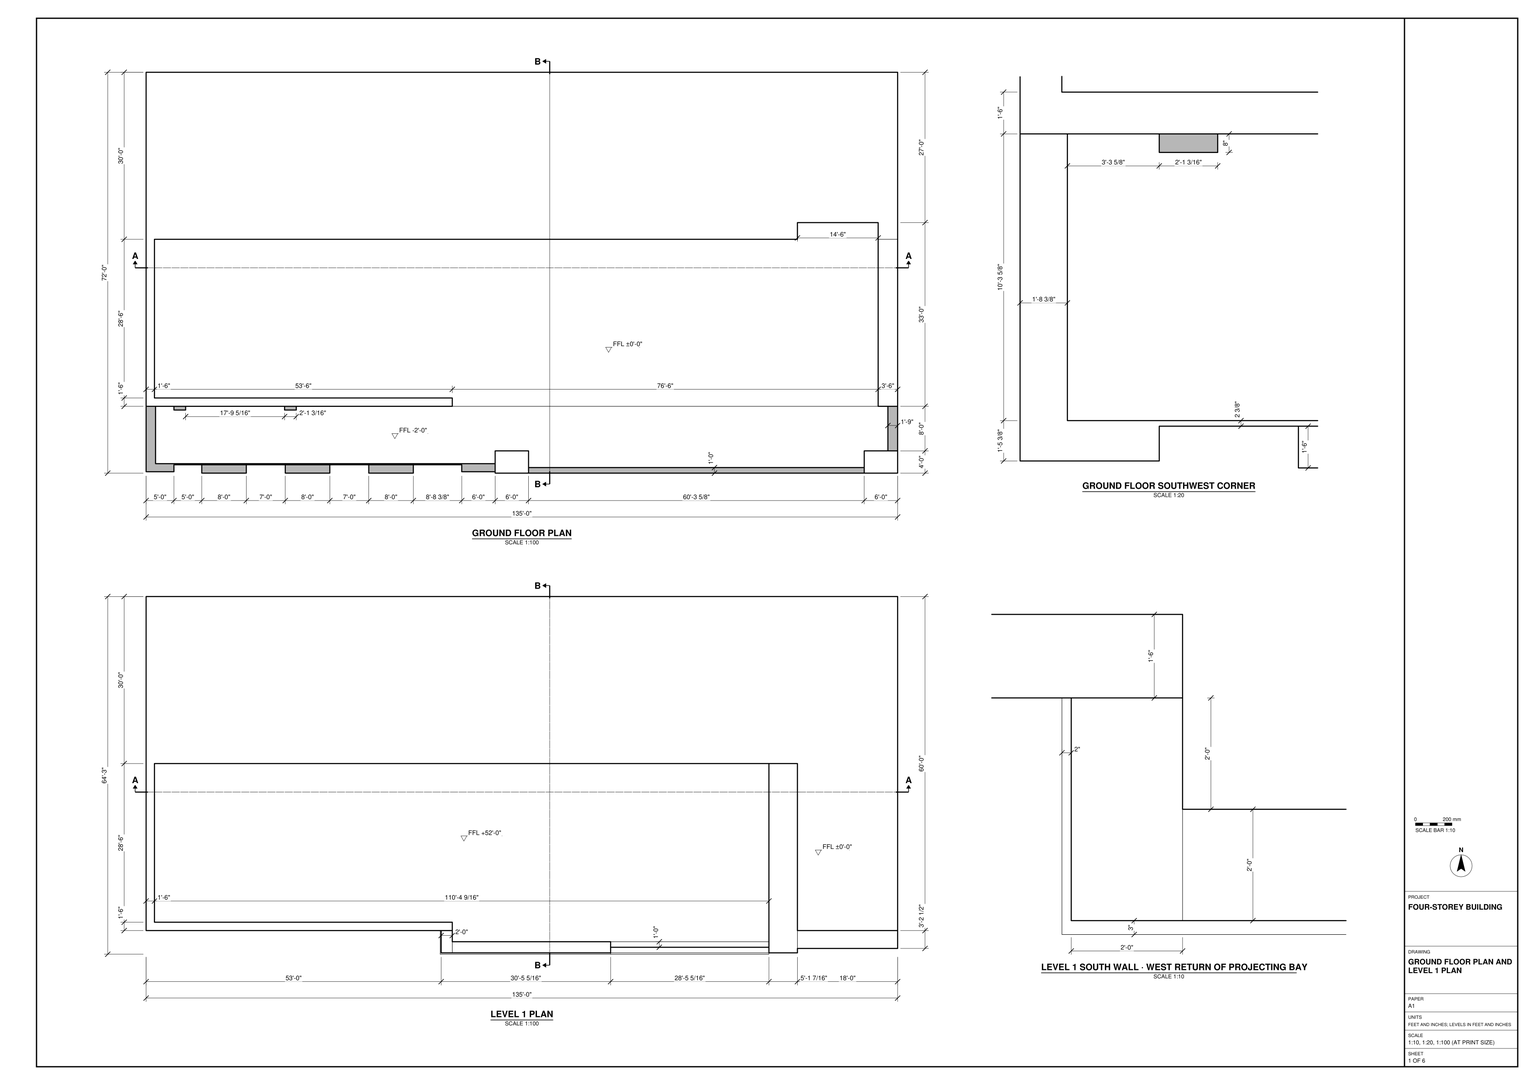
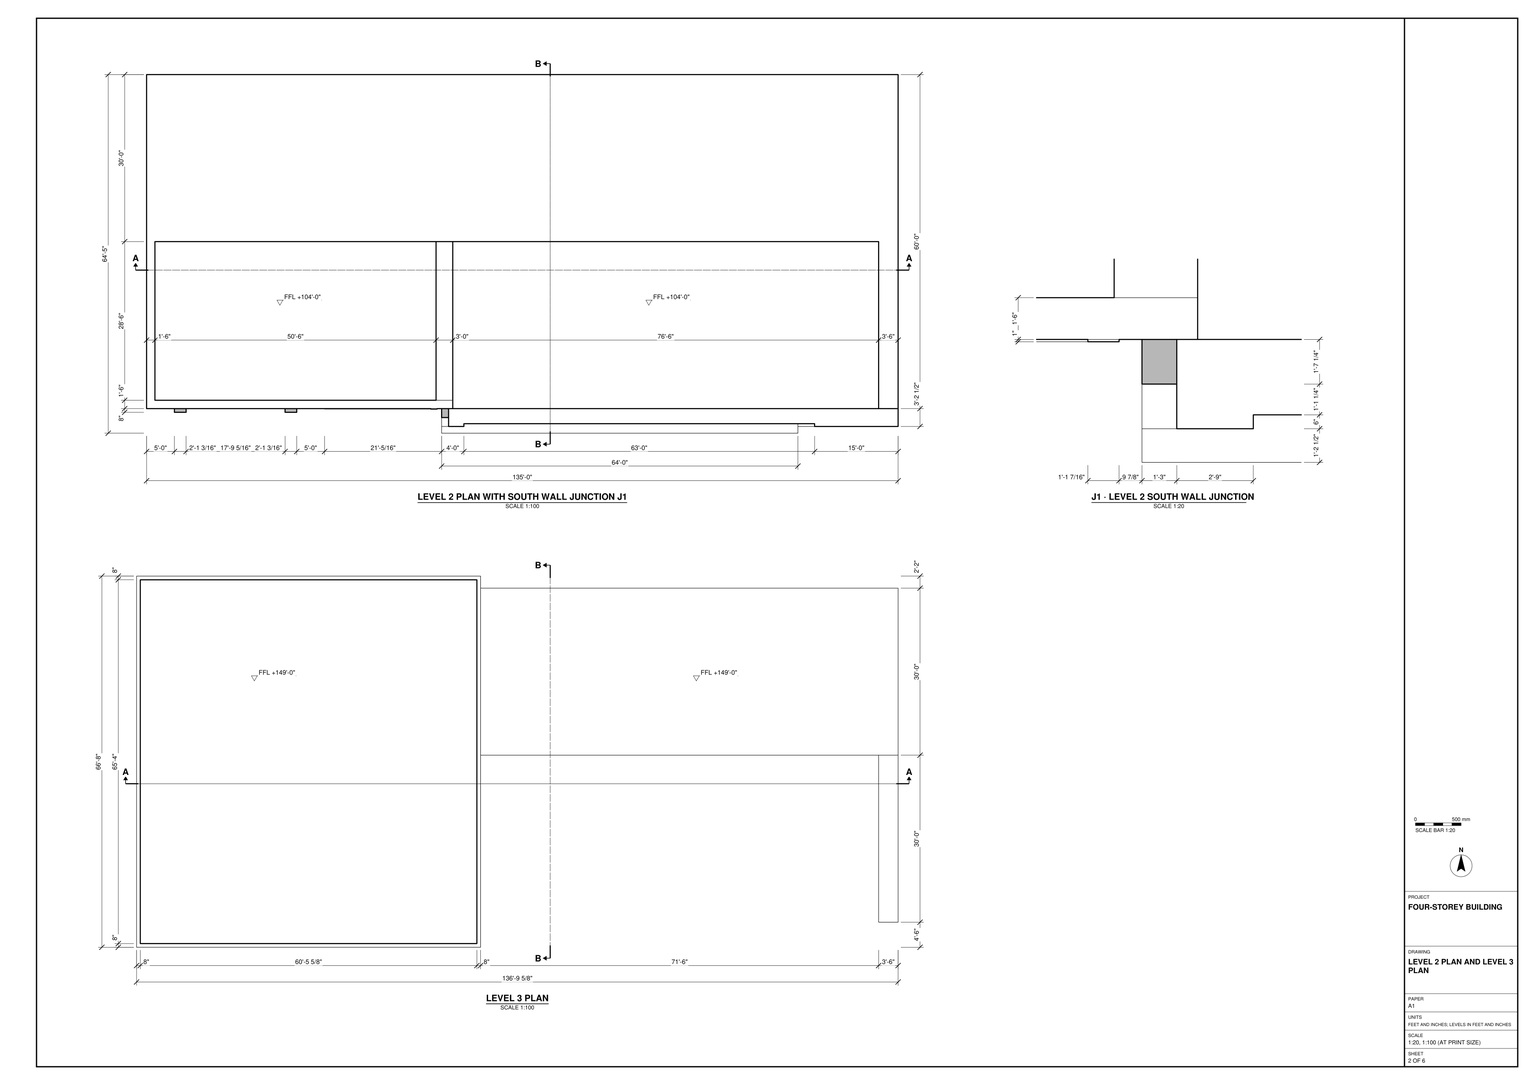
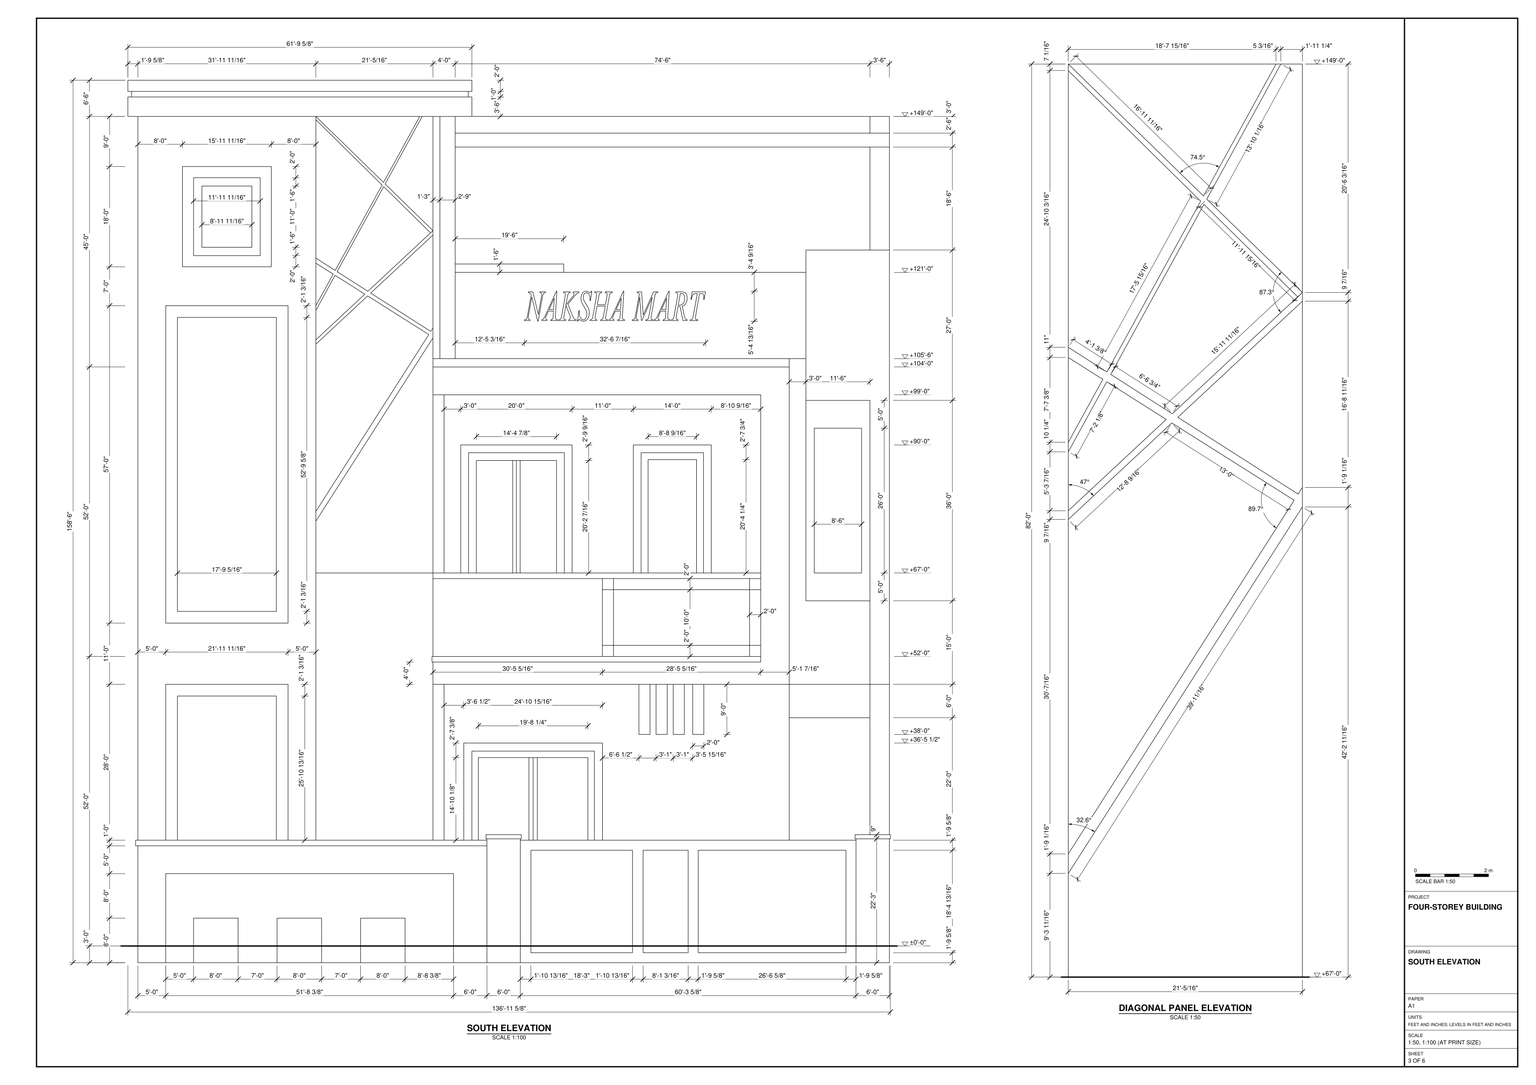
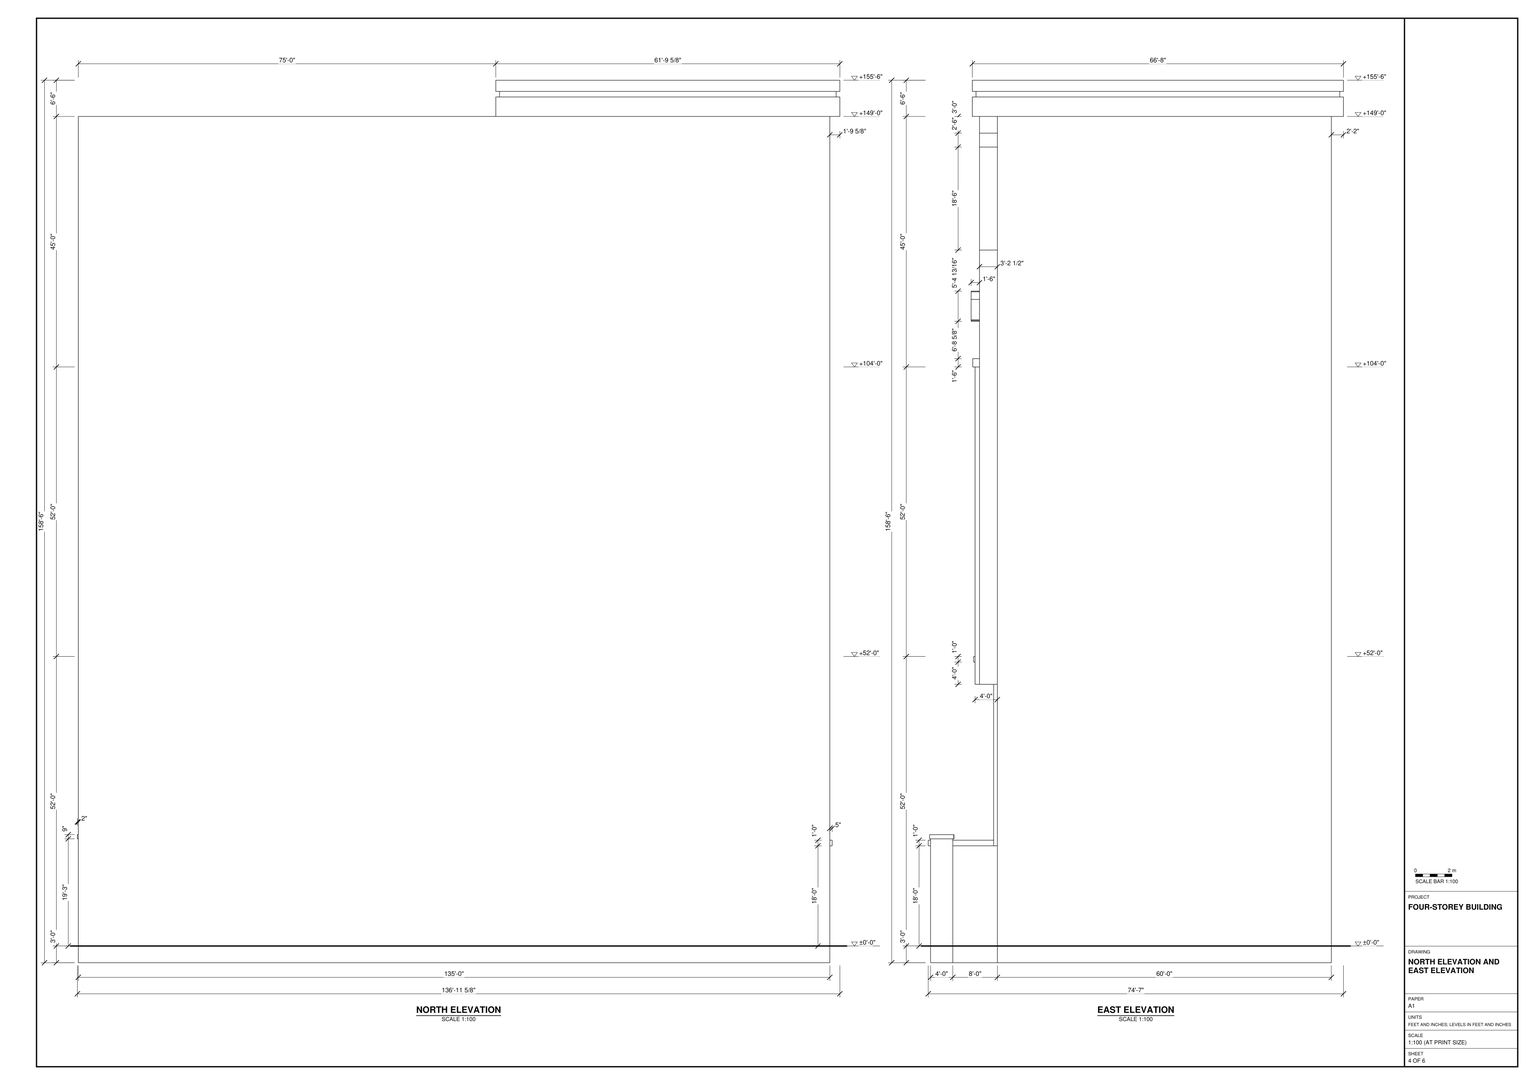
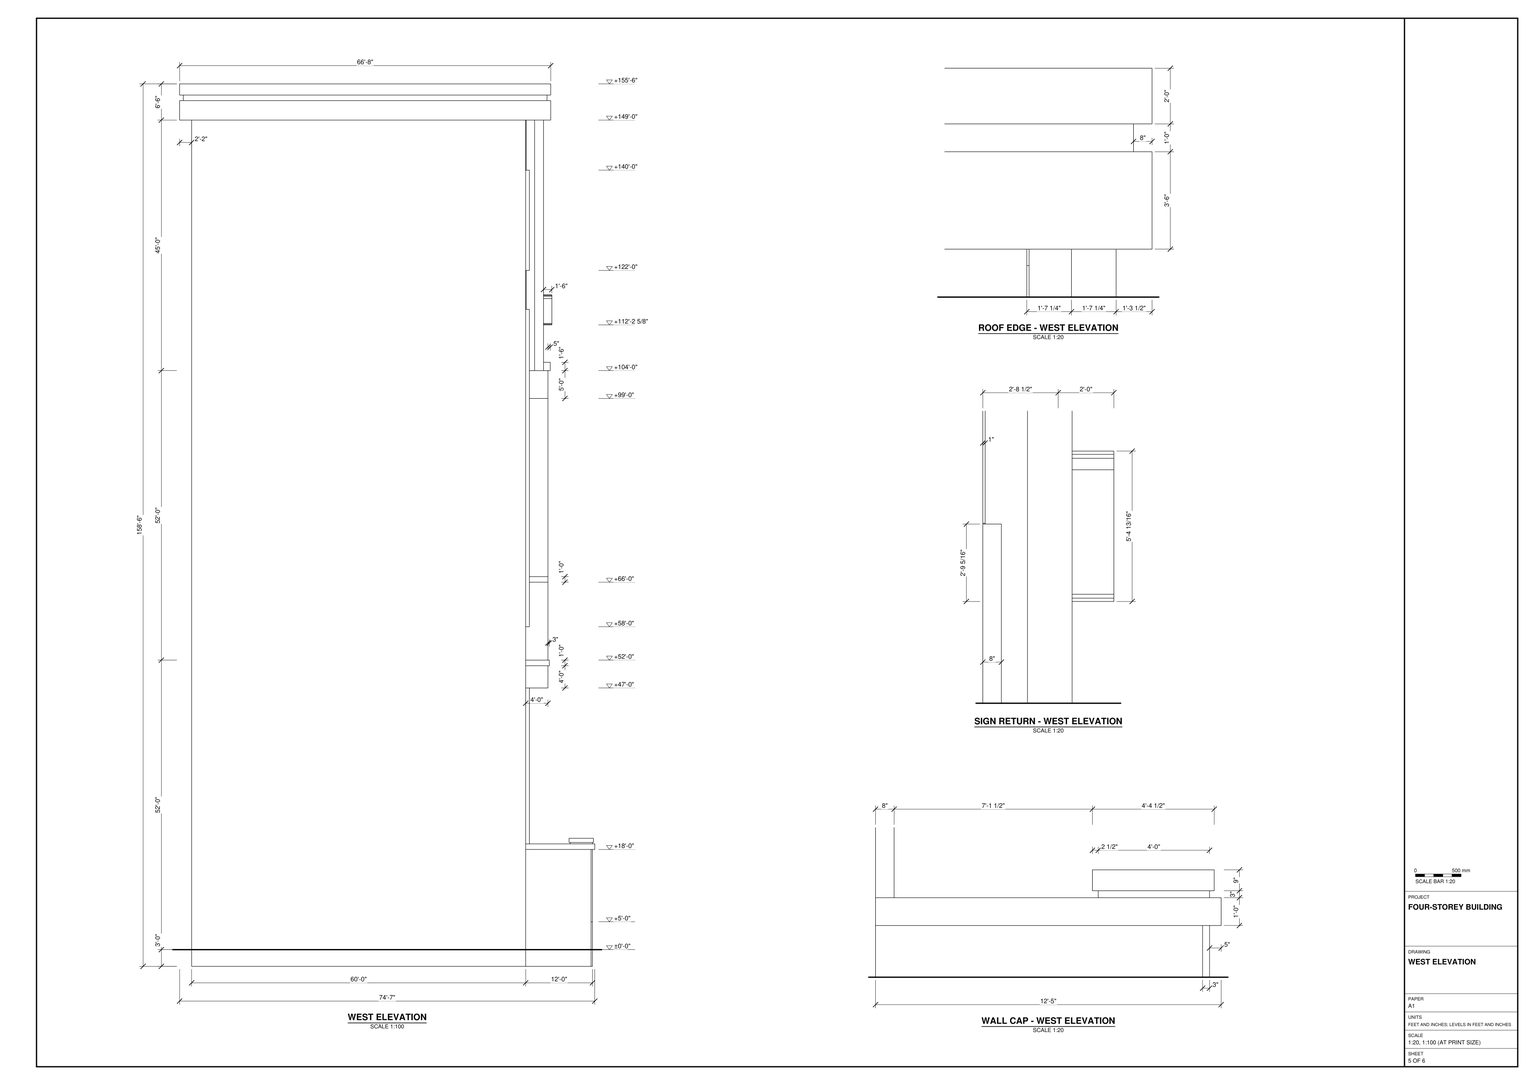
Build the four-storey building in SketchUp from task_files/diagram_01.pdf. Work in feet and inches. The overall model must measure 136'-11 5/8" east to west, 74'-7" north to south and 158'-6" high. Set the ground floor at ±0'-0" and the successive levels at +52'-0", +104'-0" and +149'-0".

Follow each floor plan separately: the slab edges and south wall change position between levels. Model the walls to their drawn thicknesses, using the enlarged details for the southwest corner, the west return of the projecting bay and the upper south wall junction. On the south elevation, form the stacked framed openings at the west, the adjacent panel with intersecting diagonal strips, and the projecting bay with its divided front and framed openings behind it. Include the entrance below the bay, the short vertical fins beside it, the sign panel above the bay and the narrow framed panel at the east. Model the low front wall with its piers and rectangular bays. Finish the roof with the raised, banded cap over the western portion and the horizontal edge extending east.

Keep walls, slabs and roof elements in separate groups or components. Group each furniture or joinery piece separately if shown, and use components for repeated parts. Any decor or loose items shown may be suitable library components. Save one SketchUp model as output_files/four_storey_building_with_its_projecting_south_bay.skp.

# SketchUp Ruby script. Lengths in inches.
U = 1.inch
M = Sketchup.active_model
def pt(a) = Geom::Point3d.new(a.map { |v| v * U })
def face(e, loops, mat)
  f = e.add_face(loops[0].map { |a| pt(a) })
  loops[1..].each { |l| e.add_face(l.map { |a| pt(a) }).erase! }
  f.material = f.back_material = mat if mat
  f
end
# faces: each face lists its corners as indices into pts; further lists are holes
def faces(e, pts, list, mat = nil) = list.each { |f| face(e, (f[0].is_a?(Array) ? f : [f]).map { |l| l.map { |i| pts[i] } }, mat) }
# xy, xz, yz: faces in a plane at the given z, y or x. An outline is a flat list of corners, or four numbers for a rectangle; further outlines are holes
def ring(l) = l.size == 4 ? [[l[0], l[1]], [l[2], l[1]], [l[2], l[3]], [l[0], l[3]]] : l.each_slice(2).to_a
def flat(e, list, mat, &to3) = list.each { |f| face(e, (f[0].is_a?(Array) ? f : [f]).map { |l| ring(l).map { |u, v| to3.(u, v) } }, mat) }
def xy(e, z, list, mat = nil) = flat(e, list, mat) { |x, y| [x, y, z] }
def xz(e, y, list, mat = nil) = flat(e, list, mat) { |x, z| [x, y, z] }
def yz(e, x, list, mat = nil) = flat(e, list, mat) { |y, z| [x, y, z] }
def lines(e, pts, list) = list.each { |a, b| e.add_line(pt(pts[a]), pt(pts[b])) }
# prism: a flat outline (further loops are holes) pulled along v
def prism(e, loops, v, mat = nil)
  f = face(e, loops, mat); d = Geom::Vector3d.new(v.map { |x| x * U })
  f.pushpull(f.normal.samedirection?(d) ? d.length : -d.length)
end
def box(e, o, s, mat = nil) = prism(e, [[o, [o[0] + s[0], o[1], o[2]], [o[0] + s[0], o[1] + s[1], o[2]], [o[0], o[1] + s[1], o[2]]]], [0, 0, s[2]], mat)
def at(x, y, z, deg = 0) = Geom::Transformation.translation(pt([x, y, z])) * Geom::Transformation.rotation(ORIGIN, Z_AXIS, deg.degrees)
def axes(o, x, y, z) = Geom::Transformation.new([*x, 0, *y, 0, *z, 0, *pt(o).to_a, 1])
def part(name) = M.definitions.add(name)
# library, detail: a bought-in or finely detailed component or shape, given as its bounding box
def library(name, o, s) = part(name).tap { |d| box(d.entities, o, s) }
def detail(e, o, s) = box(e.add_group.entities, o, s)
def put(e, d, t, mat = nil) = e.add_instance(d, t).tap { |i| i.material = mat if mat }
def group(e, t, mat = nil) = e.add_group.tap { |g| g.transformation = t; g.material = mat if mat }.entities
root = M.entities
M.materials.add("[0009_Linen]").color = [250, 240, 230]
M.materials.add("[0011_Seashell]").color = [214, 205, 199]
M.materials.add("[0011_Seashell]1").color = [221, 213, 207]
M.materials.add("[0011_Seashell]2").color = [219, 210, 204]
M.materials.add("[0013_LightCoral]").color = [255, 136, 136]
M.materials.add("[0013_LightCoral]1").color = [240, 128, 128]
M.materials.add("[0021_DarkRed]").color = [66, 0, 0]
M.materials.add("[0021_DarkRed]1").color = [43, 0, 0]
M.materials.add("[0097_DeepSkyBlue]").color = [0, 191, 255]
M.materials.add("[0133_Gray]").color = [128, 128, 128]
M.materials.add("[0136_Charcoal]").color = [35, 35, 35]
M.materials.add("[0137_Black]").color = [33, 33, 33]
M.materials.add("[0137_Black]1").color = [30, 30, 30]
M.materials.add("[Cladding Siding Tan]").color = [204, 97, 57]
M.materials.add("[Cladding Stucco White]").color = [211, 211, 211]
M.materials.add("[Granite Brown]").color = [126, 104, 91]
M.materials.add("[Granite Dark Gray]").color = [69, 68, 68]
M.materials.add("[Granite Dark Gray]1").color = [69, 68, 68]
M.materials.add("[Translucent Glass Blue]").color = [100, 149, 237]
M.materials["[Translucent Glass Blue]"].alpha = 0.5
M.materials.add("[Translucent Glass Gray]").color = [128, 128, 128]
M.materials["[Translucent Glass Gray]"].alpha = 0.5
M.materials.add("[Translucent Glass Tinted]").color = [8, 201, 241]
M.materials["[Translucent Glass Tinted]"].alpha = 0.48
M.materials.add("[White Tile Black Accent]").color = [110, 110, 110]
M.materials.add("[Wood Cherry Original]").color = [127, 72, 35]
M.materials.add("[Wood Cherry Original]1").color = [130, 73, 35]
M.materials.add("[Wood Veneer 01]").color = [120, 70, 37]
c1 = part("NAKSHA MART")
prism(c1.entities,[[[14.86,35.11,0],[25.47,8.2,0],[31.22,28.3,0],[31.92,32.15,0],[31.76,32.99,0],[31.27,33.62,0],[30.32,34.02,0],[28.81,34.15,0],[28.18,34.18,0],[28.46,35.11,0],[39.49,35.11,0],[39.19,34.18,0],[36.63,33.82,0],[35.59,33.22,0],[34.86,32.46,0],[34.04,30.82,0],[33.22,28.3,0],[25.14,0,0],[24.23,0,0],[12.81,28.96,0],[6.71,7.57,0],[6.03,3.85,0],[6.18,3,0],[6.65,2.39,0],[7.69,1.98,0],[9.59,1.72,0],[9.34,0.78,0],[-1.44,0.78,0],[-1.09,1.72,0],[1.62,2.08,0],[2.53,2.6,0],[3.16,3.27,0],[3.94,4.9,0],[4.81,7.57,0],[11.62,31.44,0],[10.6,32.72,0],[9.51,33.53,0],[8.07,33.98,0],[6,34.18,0],[6.28,35.11,0]]],[0,0,24])
prism(c1.entities,[[[61.29,35.9,0],[58.68,7.34,0],[58.48,4.71,0],[58.86,3.16,0],[60.16,2.08,0],[62.9375,1.72,0],[62.66,0.78,0],[49.14,0.78,0],[49.42,1.72,0],[50,1.72,0],[51.49,1.9,0],[52.68,2.43,0],[53.34,3.07,0],[53.82,4.03,0],[54.35,7.72,0],[54.76,12.08,0],[44.9375,12.08,0],[41.44,7.34,0],[39.95,5.05,0],[39.65,3.75,0],[39.81,2.99,0],[40.3,2.35,0],[41.18,1.91,0],[42.48,1.72,0],[42.2,0.78,0],[32.05,0.78,0],[32.33,1.72,0],[34.09,2.07,0],[35.63,2.97,0],[37.41,4.82,0],[39.9,8,0],[60.41,35.9,0]],[[56.28,27.47,0],[46.33,13.92,0],[54.96,13.92,0]]],[0,0,24])
prism(c1.entities,[[[82.81,20.3,0],[91.32,7.16,0],[93.4,4.3,0],[95.09,2.7,0],[96.82,1.97,0],[99.01,1.72,0],[98.73,0.78,0],[84.1,0.78,0],[84.33,1.72,0],[85.82,2.02,0],[86.8,2.56,0],[87.34,3.26,0],[87.52,4.05,0],[87.27,5.52,0],[85.8,8,0],[78.84,18.91,0],[75.47,7.54,0],[74.63,3.875,0],[74.81,3.03,0],[75.34,2.41,0],[76.57,1.98,0],[78.84,1.72,0],[78.43,0.78,0],[64.86,0.78,0],[65.19,1.72,0],[67.85,2.08,0],[69.34,3.24,0],[70.96,7.54,0],[77.01,28.28,0],[77.7,32.1,0],[77.53,32.99,0],[77.05,33.65,0],[76.1,34.04,0],[74.53,34.18,0],[74.03,34.18,0],[74.33,35.11,0],[87.22,35.11,0],[86.96,34.18,0],[84.58,33.82,0],[83.64,33.22,0],[82.99,32.46,0],[81.49,28.28,0],[78.84,19.47,0],[91.04,28.66,0],[93.05,30.29,0],[94.23,31.54,0],[94.68,32.73,0],[94.22,33.62,0],[92.78,34.18,0],[93.04,35.11,0],[104.03,35.11,0],[103.8,34.18,0],[100.77,33.38,0],[98.25,32.03,0],[93.32,28.28,0]]],[0,0,24])
prism(c1.entities,[[[101.19,0,0],[104.03,12.73,0],[104.89,12.73,0],[104.71,9.67,0],[104.85,8.02,0],[105.26,6.53,0],[105.95,5.19,0],[106.92,4.03,0],[108.12,3.07,0],[109.48,2.39,0],[111.01,1.98,0],[112.71,1.85,0],[114.27,1.98,0],[115.625,2.36,0],[116.79,2.99,0],[117.75,3.89,0],[119.04,6.08,0],[119.47,8.58,0],[119.27,10.23,0],[118.68,11.72,0],[116.5,14.62,0],[112.33,19.11,0],[109.11,22.89,0],[108.24,24.99,0],[107.95,27.19,0],[108.12,28.92,0],[108.62,30.53,0],[109.46,32,0],[110.63,33.34,0],[112.07,34.46,0],[113.7,35.26,0],[115.51,35.74,0],[117.52,35.9,0],[120.2,35.62,0],[123.0625,34.61,0],[124.68,33.97,0],[125.47,33.9,0],[126.73,34.28,0],[127.97,35.9,0],[128.9375,35.9,0],[126.3,24.51,0],[125.44,24.51,0],[125.54,26.96,0],[125.42,28.42,0],[125.04,29.75,0],[124.41,30.93,0],[123.52,31.97,0],[122.43,32.83,0],[121.17,33.4375,0],[118.18,33.92,0],[115.79,33.54,0],[113.9,32.38,0],[112.66,30.72,0],[112.25,28.81,0],[112.52,27.08,0],[113.3,25.43,0],[115.04,23.32,0],[118.14,20.19,0],[121.26,16.96,0],[123.04,14.52,0],[123.875,12.41,0],[124.15,10.18,0],[123.81,7.61,0],[122.77,5.125,0],[121.09,2.96,0],[118.81,1.34,0],[116.11,0.34,0],[113.16,0,0],[110.33,0.28,0],[106.125,1.65,0],[104.48,2.03,0],[103.15,1.52,0],[102.15,0,0]]],[0,0,24])
prism(c1.entities,[[[139.54,19.8,0],[155.39,19.8,0],[157.9,28.28,0],[158.61,32.125,0],[158.29,33.25,0],[157.32,33.95,0],[154.73,34.18,0],[154.99,35.11,0],[168.81,35.11,0],[168.51,34.18,0],[165.9,33.82,0],[164.84,33.22,0],[164.1,32.46,0],[163.26,30.82,0],[162.41,28.28,0],[156.35,7.54,0],[155.59,3.85,0],[155.76,3,0],[156.27,2.39,0],[157.4,1.98,0],[159.47,1.72,0],[159.19,0.78,0],[145.82,0.78,0],[146.18,1.72,0],[148.81,2.08,0],[149.68,2.59,0],[150.28,3.24,0],[151.9,7.54,0],[154.99,18.05,0],[139.0625,18.05,0],[135.95,7.54,0],[135.22,3.85,0],[135.38,3,0],[135.875,2.39,0],[137,1.98,0],[139.0625,1.72,0],[138.86,0.78,0],[125.39,0.78,0],[125.72,1.72,0],[128.38,2.08,0],[129.875,3.24,0],[131.49,7.54,0],[137.57,28.28,0],[138.3,32.125,0],[137.99,33.25,0],[137,33.95,0],[134.38,34.18,0],[134.68,35.11,0],[148.23,35.11,0],[147.95,34.18,0],[145.44,33.82,0],[144.41,33.23,0],[143.7,32.48,0],[142.9,30.875,0],[142.03,28.28,0]]],[0,0,24])
prism(c1.entities,[[[190.91,35.9,0],[188.3,7.34,0],[188.1,4.71,0],[188.48,3.16,0],[189.78,2.08,0],[192.56,1.72,0],[192.28,0.78,0],[178.76,0.78,0],[179.04,1.72,0],[179.62,1.72,0],[181.11,1.9,0],[182.3,2.43,0],[182.96,3.07,0],[183.44,4.03,0],[183.97,7.72,0],[184.38,12.08,0],[174.56,12.08,0],[171.0625,7.34,0],[169.57,5.05,0],[169.27,3.75,0],[169.43,2.99,0],[169.92,2.35,0],[170.8,1.91,0],[172.1,1.72,0],[171.82,0.78,0],[161.67,0.78,0],[161.95,1.72,0],[163.71,2.07,0],[165.25,2.97,0],[167.03,4.82,0],[169.52,8,0],[190.03,35.9,0]],[[185.9,27.47,0],[175.95,13.92,0],[184.58,13.92,0]]],[0,0,24])
prism(c1.entities,[[[225.27,35.11,0],[228.43,7.47,0],[248.35,35.11,0],[256.73,35.11,0],[256.73,34.18,0],[253.52,33.82,0],[252.72,33.33,0],[251.99,32.51,0],[251.26,31.0625,0],[250.48,28.71,0],[244.125,6.9375,0],[243.57,3.95,0],[243.74,3.08,0],[244.25,2.46,0],[245.49,1.91,0],[247.29,1.72,0],[247.9,1.72,0],[247.67,0.78,0],[233.22,0.78,0],[233.47,1.72,0],[234.15,1.72,0],[235.85,1.86,0],[237.09,2.28,0],[237.83,2.86,0],[238.49,3.81,0],[240.23,8.81,0],[245.9,28.71,0],[225.875,0.78,0],[224.86,0.78,0],[221.65,28.71,0],[215.52,7.47,0],[214.73,3.82,0],[214.91,3,0],[215.42,2.39,0],[216.59,1.98,0],[218.73,1.72,0],[218.46,0.78,0],[207.14,0.78,0],[207.42,1.72,0],[208.1,1.72,0],[210.26,2.04,0],[211.72,2.99,0],[212.55,4.43,0],[213.42,6.9375,0],[220.89,32.53,0],[219.29,33.7,0],[216.48,34.18,0],[216.73,35.11,0]]],[0,0,24])
prism(c1.entities,[[[278.73,35.9,0],[276.125,7.34,0],[275.92,4.71,0],[276.3,3.16,0],[277.61,2.08,0],[280.38,1.72,0],[280.1,0.78,0],[266.58,0.78,0],[266.86,1.72,0],[267.44,1.72,0],[268.9375,1.9,0],[270.125,2.43,0],[270.78,3.07,0],[271.27,4.03,0],[271.8,7.72,0],[272.2,12.08,0],[262.38,12.08,0],[258.89,7.34,0],[257.39,5.05,0],[257.09,3.75,0],[257.25,2.99,0],[257.75,2.35,0],[258.62,1.91,0],[259.92,1.72,0],[259.65,0.78,0],[249.49,0.78,0],[249.77,1.72,0],[251.53,2.07,0],[253.08,2.97,0],[254.86,4.82,0],[257.34,8,0],[277.85,35.9,0]],[[273.72,27.47,0],[263.77,13.92,0],[272.41,13.92,0]]],[0,0,24])
prism(c1.entities,[[[305.24,0.78,0],[299.75,17.47,0],[295.8,17.85,0],[292.84,7.47,0],[292.25,4.05,0],[292.4375,3.1,0],[292.99,2.38,0],[294.03,1.99,0],[296.03,1.72,0],[295.8,0.78,0],[282.51,0.78,0],[282.78,1.72,0],[285.32,2.1,0],[286.22,2.61,0],[286.84,3.27,0],[287.66,4.91,0],[288.53,7.47,0],[294.53,28.2,0],[295.14,31.42,0],[294.9,32.49,0],[294.19,33.39,0],[293.03,33.99,0],[291.47,34.18,0],[291.77,35.11,0],[302.96,35.11,0],[305.58,34.98,0],[307.8,34.58,0],[309.625,33.92,0],[311.0625,32.99,0],[312.15,31.84,0],[312.92,30.53,0],[313.39,29.04,0],[313.54,27.39,0],[313.39,25.77,0],[312.91,24.22,0],[312.11,22.74,0],[311,21.33,0],[309.61,20.08,0],[307.98,19.09,0],[306.12,18.34,0],[304.03,17.85,0],[307.37,7.8,0],[308.58,4.75,0],[309.8,2.99,0],[311.39,2.11,0],[313.72,1.72,0],[313.44,0.78,0]],[[296.23,19.29,0],[299.11,19.0625,0],[301.18,19.21,0],[303.01,19.67,0],[304.62,20.42,0],[306,21.48,0],[307.11,22.76,0],[307.9,24.19,0],[308.375,25.77,0],[308.53,27.49,0],[308.14,29.97,0],[306.95,31.8,0],[304.97,32.92,0],[302.2,33.29,0],[300.28,33.09,0]]],[0,0,24])
prism(c1.entities,[[[322.96,35.11,0],[349.04,35.11,0],[346.23,26,0],[345.27,26,0],[345.75,29.57,0],[345.46,31.19,0],[344.61,32.35,0],[343.07,32.89,0],[340.18,33.0625,0],[337.47,33.0625,0],[330.68,9.42,0],[329.39,3.92,0],[329.59,3.05,0],[330.2,2.34,0],[331.32,1.875,0],[333.0625,1.72,0],[334.23,1.72,0],[333.92,0.78,0],[318.99,0.78,0],[319.27,1.72,0],[319.92,1.72,0],[321.67,1.88,0],[322.96,2.35,0],[323.66,2.96,0],[324.29,3.91,0],[325.95,8.68,0],[333.0625,33.0625,0],[331.01,33.0625,0],[328.34,32.875,0],[326.24,32.3,0],[324.6,31.375,0],[323.32,30.1,0],[322.3,28.35,0],[321.49,26,0],[320.56,26,0]]],[0,0,24])
xy(root,-12,[[774,5,774,8,702,8,702,23,81.6,23,81.6,8,21.6,8,21.6,149,1641.6,149,1641.6,5],[21.6,149,1641.6,869]])
xy(root,-12,[[141.6,5,237.6,23],[321.6,5,417.6,23],[501.6,5,597.6,23]],"[0097_DeepSkyBlue]")
xy(root,0,[[81.6,141,106.8,149],[320.09,141,345.29,149]])
xy(root,0,[[846,17,1569.6,17,1569.6,53,1620.6,53,1620.6,149,345.29,149,345.29,141,320.09,141,320.09,149,106.8,149,106.8,141,81.6,141,81.6,149,42,149,42,25.4,774,25.4,774,53,846,53]],"[Granite Dark Gray]1")
xy(root,24,[[681.6,149,1599.6,149,1599.6,545,1425.6,545,1425.6,509,39.6,509,39.6,167,681.6,167]],"[Granite Dark Gray]")
xy(root,84,[[141.6,5,237.6,23],[321.6,5,417.6,23],[501.6,5,597.6,23]],"[0097_DeepSkyBlue]")
xy(root,144,[[741.6,509,1005.6,514]])
xy(root,157.875,[[755.47,509,864.6,514],[882.6,509,991.73,514]])
xy(root,180,[[81.6,8,702,23]],"[0011_Seashell]1")
xy(root,240,[[1620.6,53,1641.6,149]],"[0011_Seashell]")
xy(root,240,[[16.6,0,16.6,149,21.6,149,21.6,8,774,8,774,0]],"[0011_Seashell]1")
xy(root,252,[[846,5,1569.6,17]],"[0009_Linen]")
xy(root,252,[[16.6,0,774,0,774,25.4,42,25.4,42,149,16.6,149]],"[0011_Seashell]1")
xy(root,255,[[[772,3,848,55.5],[774,5,846,53]],[1567.6,3,1567.6,53,1569.6,53,1569.6,5,1641.6,5,1641.6,53,1567.6,53,1567.6,55,1643.6,55,1643.6,3],[774,5,846,53],[1569.6,5,1641.6,53]])
xy(root,264,[[772,3,848,55.5],[1567.6,3,1643.6,55]])
xy(root,430.125,[[755.47,509,864.6,514],[882.6,509,991.73,514]])
xy(root,444,[[741.6,509,1005.6,514]])
xy(root,516,[[1425.6,149,1599.6,545]],"[0137_Black]")
xy(root,562.8,[[106.8,141,320.09,149]])
xy(root,588,[[81.6,141,345.29,149]])
xy(root,588,[[657.6,101,657.6,149,681.6,149,681.6,167,39.6,167,39.6,509,1425.6,509,1425.6,101]],"[0011_Seashell]")
xy(root,588,[[1425.6,110.5,1641.6,149]],"[0137_Black]")
xy(root,636,[[655.6,98,655.6,149,657.6,149,657.6,101,1364.16,101,1364.16,98]],"[Wood Cherry Original]")
xy(root,648,[[657.6,101,681.6,149],[681.6,101,1022.88,125]])
xy(root,648,[[1022.88,101,1364.16,113],[1022.88,113,1364.16,125]],"[0011_Seashell]")
xy(root,648,[[681.6,125,1364.16,125,1364.16,509,39.6,509,39.6,167,681.6,167]],"[Granite Brown]")
xy(root,648,[[655.6,98,1022.88,98,1022.88,101,657.6,101,657.6,149,655.6,149],[1022.88,98,1364.16,101]],"[Wood Cherry Original]")
xy(root,712.75,[[1106.35,509,1240.85,515]])
xy(root,720,[[81.6,141,345.29,149]])
xy(root,745.2,[[106.8,141,320.09,149]])
xy(root,768,[[1461.6,110.5,1599.6,116.5]])
xy(root,816,[[1022.88,101,1364.16,113],[1022.88,113,1364.16,125]])
xy(root,828,[[657.6,101,1364.16,101,1364.16,125,681.6,125,681.6,149,657.6,149]],"[Wood Cherry Original]")
xy(root,828,[[1479.6,110.5,1581.6,121]],"[Wood Veneer 01]")
xy(root,1087.25,[[1106.35,509,1240.85,515]])
xy(root,1140,[[1479.6,110.5,1581.6,121]],"[Wood Veneer 01]")
xy(root,1200,[[1461.6,110.5,1599.6,116.5]])
xy(root,1212,[[657.6,101,657.6,149,681.6,149,681.6,167,39.6,167,39.6,509,1364.16,509,1364.16,101]],"[0011_Seashell]")
xy(root,1272,[[657.6,101,1425.6,110.5],[657.6,110.5,672.6,129.75],[657.6,129.75,672.6,149],[39.6,167,645.6,509],[645.6,167,681.6,509]])
xy(root,1272,[[681.6,149,1599.6,509]],"[Granite Brown]")
xy(root,1272,[[657.6,96,1425.6,101]],"[Wood Veneer 01]")
xy(root,1290,[[1425.6,110.5,1461.6,116.5]],"[0136_Charcoal]")
xy(root,1290,[[657.6,96,1425.6,96,1425.6,116.5,705.6,116.5,705.6,110.5,657.6,110.5]],"[Wood Veneer 01]")
xy(root,1378.8,[[106.8,141,320.09,149]])
xy(root,1404,[[81.6,141,345.29,149]])
xy(root,1476,[[705.6,116.5,939.6,149]])
xy(root,1476,[[939.6,116.5,1461.6,149]],"[0137_Black]")
xy(root,1476,[[705.6,110.5,939.6,116.5]],"[Wood Veneer 01]")
xy(root,1488,[[117.6,141,309.29,149]],"[Wood Veneer 01]")
xy(root,1494,[[705.6,110.5,939.6,149]],"[Wood Veneer 01]")
xy(root,1512,[[141.6,141,285.29,149]],"[Wood Veneer 01]")
xy(root,1524,[[1461.6,110.5,1641.6,149]],"[0013_LightCoral]")
xy(root,1680,[[141.6,141,285.29,149]],"[Wood Veneer 01]")
xy(root,1704,[[117.6,141,309.29,149]],"[Wood Veneer 01]")
xy(root,1746,[[705.6,110.5,1641.6,149],[747.6,149,778.8,509],[838.8,149,870,509],[930,149,961.2,509],[1021.2,149,1052.4,509],
  [1112.4,149,1143.6,509],[1203.6,149,1234.8,509],[1294.8,149,1326,509],[1386,149,1417.2,509],[1477.2,149,1508.4,509],
  [1568.4,149,1599.6,509]],"[Wood Veneer 01]")
xy(root,1776,[[705.6,110.5,1641.6,149],[747.6,149,778.8,509],[838.8,149,870,509],[930,149,961.2,509],[1021.2,149,1052.4,509],
  [1112.4,149,1143.6,509],[1203.6,149,1234.8,509],[1294.8,149,1326,509],[1386,149,1417.2,509],[1477.2,149,1508.4,509],
  [1568.4,149,1599.6,509]],"[Wood Veneer 01]")
xy(root,1794,[[681.6,149,705.6,509]],"[Wood Veneer 01]")
xy(root,1812,[[672.6,110.5,705.6,149],[657.6,129.75,672.6,149],[629.2,148,629.2,149,21.6,149,21.6,509,39.6,509,39.6,167,681.6,167,681.6,149,634.37,149,634.37,148],[681.6,149,705.6,167],[39.6,167,645.6,509],
  [645.6,167,681.6,509],[681.6,167,705.6,509],[21.6,509,741.6,869]])
xy(root,1812,[[1599.6,149,1641.6,509],[741.6,509,1641.6,869]],"[0011_Seashell]")
xy(root,1812,[[0,95,0,895,741.6,895,741.6,869,21.6,869,21.6,149,629.2,149,629.2,148,634.37,148,634.37,149,657.6,149,657.6,129.75,672.6,129.75,672.6,110.5,705.6,110.5,705.6,509,741.6,509,741.6,95]],"[0011_Seashell]2")
xy(root,1854,[[8,103,733.6,887]])
xy(root,1854,[[[0,95,741.6,895],[8,103,733.6,887]]],"[0011_Seashell]2")
xy(root,1866,[[8,103,733.6,887]])
xy(root,1866,[[[0,95,741.6,895],[8,103,733.6,887]]],"[0011_Seashell]2")
xy(root,1890,[[0,95,741.6,895]],"[0011_Seashell]2")
xz(root,0,[[16.6,240,774,252]],"[0011_Seashell]1")
xz(root,3,[[772,255,848,264],[1567.6,255,1643.6,264]])
xz(root,5,[[774,-12,846,255],[1569.6,-12,1641.6,255]])
xz(root,5,[[141.6,-12,237.6,84],[321.6,-12,417.6,84],[501.6,-12,597.6,84],[868.8,9.6,1087.8,230.4],[1110.6,9.6,1207.8,230.4]],"[0097_DeepSkyBlue]")
xz(root,5,[[[846,-12,1569.6,252],[1229.4,9.6,1548,230.4],[868.8,9.6,1087.8,230.4],[1110.6,9.6,1207.8,230.4]]],"[0137_Black]1")
xz(root,5,[[1229.4,9.6,1548,230.4]],"[Cladding Siding Tan]")
xz(root,8,[[21.6,-12,81.6,-12,81.6,180,702,180,702,-12,774,-12,774,240,21.6,240]],"[0011_Seashell]1")
xz(root,17,[[846,0,1569.6,252]],"[0009_Linen]")
xz(root,23,[[81.6,-12,141.6,-12,141.6,84,237.6,84,237.6,-12,321.6,-12,321.6,84,417.6,84,417.6,-12,501.6,-12,501.6,84,597.6,84,597.6,-12,702,-12,702,180,81.6,180],[141.6,-12,237.6,84],[321.6,-12,417.6,84],[501.6,-12,597.6,84]])
xz(root,25.4,[[42,0,774,252]],"[0011_Seashell]1")
xz(root,53,[[774,0,846,255],[1569.6,0,1569.6,255,1641.6,255,1641.6,240,1620.6,240,1620.6,0],[1620.6,0,1641.6,240]])
xz(root,55,[[1567.6,255,1643.6,264]])
xz(root,55.5,[[772,255,848,264]])
xz(root,95,[[0,1812,741.6,1854],[0,1866,741.6,1890]],"[0011_Seashell]2")
xz(root,96,[[657.6,1272,1425.6,1290]],"[Wood Veneer 01]")
xz(root,98,[[655.6,636,1364.16,648]],"[Wood Cherry Original]")
xz(root,101,[[657.6,636,1364.16,648]])
xz(root,101,[[657.6,588,1425.6,588,1425.6,1272,657.6,1272,657.6,1212,1364.16,1212,1364.16,636,657.6,636],[657.6,648,1022.88,816]],"[0011_Seashell]")
xz(root,101,[[657.6,816,1364.16,828]],"[Wood Cherry Original]")
xz(root,103,[[8,1854,733.6,1866]],"[0133_Gray]")
xz(root,110.5,[[1599.6,588,1641.6,588,1641.6,1524,1461.6,1524,1461.6,1200,1599.6,1200]],"[0013_LightCoral]")
xz(root,110.5,[[1425.6,588,1599.6,588,1599.6,768,1461.6,768,1461.6,1290,1425.6,1290]],"[0137_Black]")
xz(root,110.5,[[[1461.6,768,1599.6,1200],[1479.6,828,1581.6,1140]],[657.6,1272,672.6,1290],[672.6,1290,705.6,1812],[705.6,1476,939.6,1494],[705.6,1746,1641.6,1776]],"[Wood Veneer 01]")
xz(root,113,[[1046.88,648,1340.16,672]],"[0011_Seashell]")
xz(root,113,[[1022.88,648,1046.88,672],[1340.16,648,1364.16,672],[1022.88,672,1046.88,792],[1046.88,672,1340.16,792],[1340.16,672,1364.16,792],
  [1022.88,792,1046.88,816],[1046.88,792,1340.16,816],[1340.16,792,1364.16,816]],"[Translucent Glass Gray]")
xz(root,116.5,[[1461.6,768,1461.6,1476,705.6,1476,705.6,1290,1461.6,1290,1461.6,1200,1599.6,1200,1599.6,768]],"[Cladding Stucco White]")
xz(root,121,[[1479.6,828,1581.6,1140]])
xz(root,125,[[1022.88,816,1364.16,828]])
xz(root,125,[[681.6,648,1022.88,828]],"[0011_Seashell]")
xz(root,129.75,[[657.6,1272,672.6,1812]])
xz(root,141,[[81.6,0,106.8,0,106.8,562.8,320.09,562.8,320.09,0,345.29,0,345.29,588,81.6,588],[[81.6,720,345.29,1404],[106.8,745.2,320.09,1378.8]]])
xz(root,141,[[[117.6,1488,309.29,1704],[141.6,1512,285.29,1680]]],"[Wood Veneer 01]")
xz(root,148,[[405.29,939.7,657.6,1334.69,657.6,1355.75,652.98,1348.52,523.39,1431.3,657.6,1556.41,657.6,1565.84,652.52,1561.11,517.39,1435.13,451.03,1477.52,551.47,1660.76,652.52,1561.11,657.6,1565.84,554.55,1666.38,634.37,1812,629.2,1812,551.08,1669.77,405.29,1812,405.29,1804.92,548,1664.18,446.92,1480.15,405.29,1506.74,405.29,1495.74,442.55,1472.19,405.29,1404.36,405.29,1394.07,446.68,1469.58,510.84,1429.03,405.29,1330.63,405.29,1321.2,516.875,1425.22,648.74,1341.88,405.29,960.75]])
xz(root,149,[[21.6,-12,1641.6,0],[21.6,0,42,252],[81.6,0,81.6,588,345.29,588,345.29,0,320.09,0,320.09,562.8,106.8,562.8,106.8,0],[106.8,0,320.09,562.8],[657.6,0,681.6,588],
  [1620.6,0,1641.6,240],[16.6,240,21.6,252],[657.6,588,681.6,624],[1425.6,588,1425.6,1272,1641.6,1272,1641.6,624,1599.6,624,1599.6,588],[1599.6,588,1641.6,624],
  [657.6,624,681.6,648],[655.6,636,657.6,648],[657.6,648,681.6,828],[[81.6,720,345.29,1404],[106.8,745.2,320.09,1378.8]],[657.6,1272,672.6,1812],
  [672.6,1272,681.6,1812],[1599.6,1272,1641.6,1524],[[117.6,1488,309.29,1704],[141.6,1512,285.29,1680]],[[141.6,1512,285.29,1680],[159.6,1530,267.29,1662]],[747.6,1746,778.8,1776],
  [838.8,1746,870,1776],[930,1746,961.2,1776],[1021.2,1746,1052.4,1776],[1112.4,1746,1143.6,1776],[1203.6,1746,1234.8,1776],
  [1294.8,1746,1326,1776],[1386,1746,1417.2,1776],[1477.2,1746,1508.4,1776],[1568.4,1746,1599.6,1776],[1599.6,1746,1641.6,1776]])
xz(root,149,[[657.6,828,681.6,1212],[1599.6,1524,1641.6,1746],[1599.6,1776,1641.6,1812]],"[0011_Seashell]")
xz(root,149,[[[42,0,81.6,0,81.6,588,345.29,588,345.29,0,405.29,0,405.29,1812,21.6,1812,21.6,252,42,252],[81.6,720,345.29,1404],[117.6,1488,309.29,1704]]],"[0011_Seashell]2")
xz(root,149,[[1599.6,0,1620.6,0,1620.6,240,1641.6,240,1641.6,588,1599.6,588]],"[0013_LightCoral]")
xz(root,149,[[1425.6,516,1599.6,588],[681.6,1272,681.6,1794,705.6,1794,705.6,1476,1461.6,1476,1461.6,1524,1599.6,1524,1599.6,1272]],"[0137_Black]")
xz(root,149,[[405.29,0,657.6,0,657.6,636,655.6,636,655.6,648,657.6,648,657.6,828,405.29,828]],"[Cladding Stucco White]")
xz(root,149,[[681.6,0,1599.6,24]],"[Granite Dark Gray]1")
xz(root,149,[[159.6,1530,267.29,1662]],"[Translucent Glass Blue]")
xz(root,149,[[405.29,828,657.6,828,657.6,1334.69,405.29,939.7],[405.29,960.75,648.74,1341.88,516.875,1425.22,405.29,1321.2],[405.29,1330.63,510.84,1429.03,446.68,1469.58,405.29,1394.07],[652.98,1348.52,657.6,1355.75,657.6,1556.41,523.39,1431.3],[405.29,1404.36,442.55,1472.19,405.29,1495.74],
  [517.39,1435.13,652.52,1561.11,551.47,1660.76,451.03,1477.52],[446.92,1480.15,548,1664.18,405.29,1804.92,405.29,1506.74],[657.6,1565.84,657.6,1812,634.37,1812,554.55,1666.38],[551.08,1669.77,629.2,1812,405.29,1812]],"[Translucent Glass Tinted]")
xz(root,149,[[106.8,745.2,320.09,1378.8]],"[White Tile Black Accent]")
xz(root,149,[[870,1746,930,1776],[961.2,1746,1021.2,1776],[1052.4,1746,1112.4,1776],[1143.6,1746,1203.6,1776],[1234.8,1746,1294.8,1776],
  [1326,1746,1386,1776],[1417.2,1746,1477.2,1776],[1508.4,1746,1568.4,1776]],"[Wood Cherry Original]1")
xz(root,149,[[705.6,1476,939.6,1494],[705.6,1746,747.6,1776],[778.8,1746,838.8,1776]],"[Wood Veneer 01]")
xz(root,167,[[39.6,1272,645.6,1812]])
xz(root,167,[[39.6,24,681.6,588],[39.6,648,681.6,1212]],"[0011_Seashell]")
xz(root,509,[[[724.125,126.52,1023.08,461.48],[741.6,144,1005.6,444]],[39.6,588,681.6,624],[681.6,588,1425.6,624],[1364.16,648,1364.16,1212,1341.6,1212,1341.6,1248,1425.6,1248,1425.6,648],[[1089.6,696,1257.6,1104],[1106.35,712.75,1240.85,1087.25]],
  [[717.6,780,957.6,1104],[734.35,796.75,940.85,1087.25]],[39.6,1272,645.6,1812],[645.6,1272,681.6,1812],[1568.4,1746,1599.6,1776],[681.6,1794,705.6,1812]])
xz(root,509,[[[39.6,24,1425.6,24,1425.6,588,1241.54,588,1241.54,480,1217.54,480,1217.54,588,1199.6,588,1199.6,480,1175.6,480,1175.6,588,1162.6,588,1162.6,480,1138.6,480,1138.6,588,1125.6,588,1125.6,480,1101.6,480,1101.6,588,39.6,588],[724.125,126.52,1023.08,461.48]],[[39.6,648,1364.16,1212],[717.6,780,957.6,1104],[1089.6,696,1257.6,1104]],[[681.6,1272,1599.6,1272,1599.6,1746,1568.4,1746,1568.4,1776,1599.6,1776,1599.6,1812,705.6,1812,705.6,1794,681.6,1794],[747.6,1746,778.8,1776],[838.8,1746,870,1776],[930,1746,961.2,1776],[1021.2,1746,1052.4,1776],[1112.4,1746,1143.6,1776],[1203.6,1746,1234.8,1776],[1294.8,1746,1326,1776],[1386,1746,1417.2,1776],[1477.2,1746,1508.4,1776]]],"[0011_Seashell]")
xz(root,509,[[[734.35,796.75,940.85,1087.25],[751.15,813.55,924.05,1070.45]],[829.6,813.55,837.6,1070.45],[837.6,813.55,845.6,1070.45]],"[0021_DarkRed]")
xz(root,509,[[1101.6,480,1125.6,588],[1138.6,480,1162.6,588],[1175.6,480,1199.6,588],[1217.54,480,1241.54,588]],"[0021_DarkRed]1")
xz(root,509,[[755.47,157.875,864.6,430.125],[882.6,157.875,991.73,430.125]],"[Translucent Glass Gray]")
xz(root,509,[[751.15,813.55,829.6,1070.45],[845.6,813.55,924.05,1070.45]],"[Translucent Glass Tinted]")
xz(root,514,[[[741.6,144,1005.6,444],[755.47,157.875,991.73,430.125]],[864.6,157.875,873.6,430.125],[873.6,157.875,882.6,430.125]],"[0021_DarkRed]")
xz(root,515,[[[1106.35,712.75,1240.85,1087.25],[1121.33,727.73,1225.87,1072.27]]],"[0021_DarkRed]")
xz(root,515,[[1121.33,727.73,1225.87,1072.27]],"[Translucent Glass Tinted]")
xz(root,545,[[1425.6,24,1599.6,516]],"[0013_LightCoral]")
xz(root,869,[[21.6,-12,1641.6,1812]],"[0011_Seashell]1")
xz(root,887,[[8,1851.6875,733.6,1854]])
xz(root,887,[[8,1854,733.6,1866]],"[0133_Gray]")
xz(root,895,[[0,1812,741.6,1854],[0,1866,741.6,1890]],"[0011_Seashell]2")
yz(root,0,[[95,1812,895,1854],[95,1866,895,1890]],"[0011_Seashell]2")
yz(root,8,[[103,1851.6875,887,1854]])
yz(root,8,[[103,1854,887,1866]],"[0133_Gray]")
yz(root,16.6,[[0,240,149,252]],"[0011_Seashell]1")
yz(root,21.6,[[8,-12,149,240],[149,-12,869,1812]],"[0011_Seashell]1")
yz(root,39.6,[[167,588,509,624],[167,1272,509,1812]])
yz(root,39.6,[[167,24,509,588],[167,648,509,1212]],"[0011_Seashell]")
yz(root,42,[[25.4,0,149,252]],"[0011_Seashell]1")
yz(root,81.6,[[141,0,149,588],[141,720,149,1404]])
yz(root,81.6,[[8,-12,23,180]],"[0011_Seashell]1")
yz(root,106.8,[[141,0,149,562.8],[141,745.2,149,1378.8]])
yz(root,117.6,[[141,1488,149,1704]],"[Wood Veneer 01]")
yz(root,141.6,[[5,-12,23,84]],"[0097_DeepSkyBlue]")
yz(root,141.6,[[141,1512,149,1680]],"[Wood Veneer 01]")
yz(root,237.6,[[5,-12,23,84]],"[0097_DeepSkyBlue]")
yz(root,285.29,[[141,1512,149,1680]],"[Wood Veneer 01]")
yz(root,309.29,[[141,1488,149,1704]],"[Wood Veneer 01]")
yz(root,320.09,[[141,0,149,562.8],[141,745.2,149,1378.8]])
yz(root,321.6,[[5,-12,23,84]],"[0097_DeepSkyBlue]")
yz(root,345.29,[[141,0,149,588],[141,720,149,1404]])
yz(root,405.29,[[148,939.7,149,960.75],[148,1321.2,149,1330.63],[148,1394.07,149,1404.36],[148,1495.74,149,1506.74],[148,1804.92,149,1812]])
yz(root,417.6,[[5,-12,23,84]],"[0097_DeepSkyBlue]")
yz(root,501.6,[[5,-12,23,84]],"[0097_DeepSkyBlue]")
yz(root,597.6,[[5,-12,23,84]],"[0097_DeepSkyBlue]")
yz(root,645.6,[[167,1272,509,1812]])
yz(root,655.6,[[98,636,149,648]],"[Wood Cherry Original]")
yz(root,657.6,[[101,588,149,636],[101,636,149,648],[101,648,149,816],[101,1212,149,1272],[129.75,1272,129.75,1812,149,1812,149,1565.84,148,1565.84,148,1556.41,149,1556.41,149,1355.75,148,1355.75,148,1334.69,149,1334.69,149,1272],
  [148,1334.69,149,1355.75],[148,1556.41,149,1565.84]])
yz(root,657.6,[[101,816,149,828]],"[Wood Cherry Original]")
yz(root,657.6,[[96,1272,110.5,1290]],"[Wood Veneer 01]")
yz(root,672.6,[[129.75,1272,149,1812]])
yz(root,672.6,[[110.5,1272,129.75,1812]],"[Wood Veneer 01]")
yz(root,681.6,[[149,588,167,624],[149,1794,509,1812]])
yz(root,681.6,[[149,24,167,588],[125,648,149,828],[149,648,167,1212],[149,1272,509,1794]],"[0011_Seashell]")
yz(root,702,[[8,-12,23,180]],"[0011_Seashell]1")
yz(root,705.6,[[110.5,1476,149,1494],[110.5,1746,149,1776]])
yz(root,705.6,[[110.5,1290,116.5,1476],[110.5,1494,149,1746],[110.5,1776,149,1776,149,1794,509,1794,509,1812,110.5,1812]],"[Wood Veneer 01]")
yz(root,733.6,[[103,1854,887,1866]],"[0133_Gray]")
yz(root,741.6,[[509,144,514,444]])
yz(root,741.6,[[95,1812,895,1854],[95,1866,895,1890]],"[0011_Seashell]2")
yz(root,747.6,[[149,1746,509,1776]],"[Wood Veneer 01]")
yz(root,755.47,[[509,157.875,514,430.125]])
yz(root,772,[[3,255,55.5,264]])
yz(root,774,[[5,-12,8,240],[25.4,0,25.4,252,5,252,5,255,53,255,53,0],[8,0,8,240,5,240,5,252,25.4,252,25.4,0]])
yz(root,774,[[0,240,5,252]],"[0011_Seashell]1")
yz(root,778.8,[[149,1746,509,1776]],"[Wood Veneer 01]")
yz(root,838.8,[[149,1746,509,1776]],"[Wood Veneer 01]")
yz(root,846,[[17,0,53,0,53,255,5,255,5,252,17,252],[5,0,17,252]])
yz(root,848,[[3,255,55.5,264]])
yz(root,864.6,[[509,157.875,514,430.125]])
yz(root,870,[[149,1746,509,1776]],"[Wood Veneer 01]")
yz(root,882.6,[[509,157.875,514,430.125]])
yz(root,930,[[149,1746,509,1776]],"[Wood Veneer 01]")
yz(root,939.6,[[110.5,1476,149,1494]],"[Wood Veneer 01]")
yz(root,961.2,[[149,1746,509,1776]],"[Wood Veneer 01]")
yz(root,991.73,[[509,157.875,514,430.125]])
yz(root,1005.6,[[509,144,514,444]])
yz(root,1021.2,[[149,1746,509,1776]],"[Wood Veneer 01]")
yz(root,1022.88,[[101,648,113,816],[113,648,125,816]],"[0011_Seashell]")
yz(root,1052.4,[[149,1746,509,1776]],"[Wood Veneer 01]")
yz(root,1106.35,[[509,712.75,515,1087.25]])
yz(root,1112.4,[[149,1746,509,1776]],"[Wood Veneer 01]")
yz(root,1143.6,[[149,1746,509,1776]],"[Wood Veneer 01]")
yz(root,1203.6,[[149,1746,509,1776]],"[Wood Veneer 01]")
yz(root,1234.8,[[149,1746,509,1776]],"[Wood Veneer 01]")
yz(root,1240.85,[[509,712.75,515,1087.25]])
yz(root,1294.8,[[149,1746,509,1776]],"[Wood Veneer 01]")
yz(root,1326,[[149,1746,509,1776]],"[Wood Veneer 01]")
yz(root,1364.16,[[98,636,101,648],[101,648,113,816]])
yz(root,1364.16,[[113,648,113,816,125,816,125,828,101,828,101,1212,509,1212,509,648]],"[0011_Seashell]")
yz(root,1386,[[149,1746,509,1776]],"[Wood Veneer 01]")
yz(root,1417.2,[[149,1746,509,1776]],"[Wood Veneer 01]")
yz(root,1425.6,[[110.5,588,149,624],[149,588,509,624],[110.5,624,149,648],[149,648,509,1248]])
yz(root,1425.6,[[101,588,110.5,1272]],"[0011_Seashell]2")
yz(root,1425.6,[[509,24,545,516]],"[0013_LightCoral]")
yz(root,1425.6,[[149,516,509,588]],"[0137_Black]")
yz(root,1425.6,[[96,1272,110.5,1290]],"[Wood Veneer 01]")
yz(root,1461.6,[[110.5,768,116.5,1200],[110.5,1200,116.5,1290]])
yz(root,1461.6,[[110.5,1290,110.5,1524,149,1524,149,1476,116.5,1476,116.5,1290]],"[0013_LightCoral]1")
yz(root,1477.2,[[149,1746,509,1776]],"[Wood Veneer 01]")
yz(root,1479.6,[[110.5,828,121,1140]],"[Wood Veneer 01]")
yz(root,1508.4,[[149,1746,509,1776]],"[Wood Veneer 01]")
yz(root,1567.6,[[3,255,55,264]])
yz(root,1568.4,[[149,1746,509,1776]],"[Wood Veneer 01]")
yz(root,1569.6,[[17,0,17,252,5,252,5,255,53,255,53,0],[5,0,17,252]])
yz(root,1581.6,[[110.5,828,121,1140]],"[Wood Veneer 01]")
yz(root,1599.6,[[149,516,509,624],[110.5,768,116.5,1200],[149,1746,509,1776]])
yz(root,1599.6,[[149,1272,509,1746]],"[0011_Seashell]")
yz(root,1599.6,[[149,1776,509,1812]],"[0011_Seashell]2")
yz(root,1599.6,[[149,24,545,516]],"[0013_LightCoral]")
yz(root,1620.6,[[53,0,149,240]],"[0011_Seashell]")
yz(root,1641.6,[[5,-12,53,255]])
yz(root,1641.6,[[53,-12,149,240],[149,-12,869,1812]],"[0011_Seashell]")
yz(root,1641.6,[[110.5,588,149,1524]],"[0013_LightCoral]")
yz(root,1641.6,[[110.5,1746,149,1776]],"[Wood Cherry Original]1")
yz(root,1643.6,[[3,255,55,264]])
p = [[405.29,149,939.7],[657.6,149,1334.69],[657.6,148,1334.69],[405.29,148,939.7],[648.74,149,1341.88],[405.29,149,960.75],
  [405.29,148,960.75],[648.74,148,1341.88],[405.29,149,1321.2],[516.875,149,1425.22],[516.875,148,1425.22],[405.29,148,1321.2],
  [510.84,149,1429.03],[405.29,149,1330.63],[405.29,148,1330.63],[510.84,148,1429.03],[652.98,149,1348.52],[523.39,149,1431.3],
  [523.39,148,1431.3],[652.98,148,1348.52],[657.6,149,1355.75],[657.6,148,1355.75],[405.29,149,1394.07],[446.68,149,1469.58],
  [446.68,148,1469.58],[405.29,148,1394.07],[442.55,149,1472.19],[405.29,149,1404.36],[405.29,148,1404.36],[442.55,148,1472.19],
  [657.6,149,1556.41],[657.6,148,1556.41],[517.39,149,1435.13],[451.03,149,1477.52],[451.03,148,1477.52],[517.39,148,1435.13],
  [652.52,149,1561.11],[652.52,148,1561.11],[405.29,149,1495.74],[405.29,148,1495.74],[551.47,149,1660.76],[551.47,148,1660.76],
  [446.92,149,1480.15],[405.29,149,1506.74],[405.29,148,1506.74],[446.92,148,1480.15],[548,149,1664.18],[548,148,1664.18],
  [657.6,149,1565.84],[554.55,149,1666.38],[554.55,148,1666.38],[657.6,148,1565.84],[405.29,149,1804.92],[405.29,148,1804.92],
  [634.37,149,1812],[634.37,148,1812],[551.08,149,1669.77],[405.29,149,1812],[405.29,148,1812],[551.08,148,1669.77],
  [629.2,149,1812],[629.2,148,1812],[1599.6,509,24],[1641.6,509,24],[1599.6,509,624],[1425.6,509,624],
  [0,103,1851.1875],[733.6,103,1851.1875],[733.6,103,1854]]
faces(root,p,[[0,1,2,3],[4,5,6,7],[8,9,10,11],[12,13,14,15],[9,4,7,10],[16,17,18,19],[20,16,19,21],[22,23,24,25],
  [26,27,28,29],[23,12,15,24],[17,30,31,18],[32,33,34,35],[36,32,35,37],[38,26,29,39],[33,40,41,34],[42,43,44,45],
  [46,42,45,47],[40,36,37,41],[48,49,50,51],[52,46,47,53],[49,54,55,50],[56,57,58,59],[60,56,59,61]])
lines(root,p,[[62,63],[64,65],[66,67],[68,67]])
put(root,c1,axes([856.42,116.5,1370.64],[1.11405,0,0],[0,0,1.80553],[0,-1,0]))
